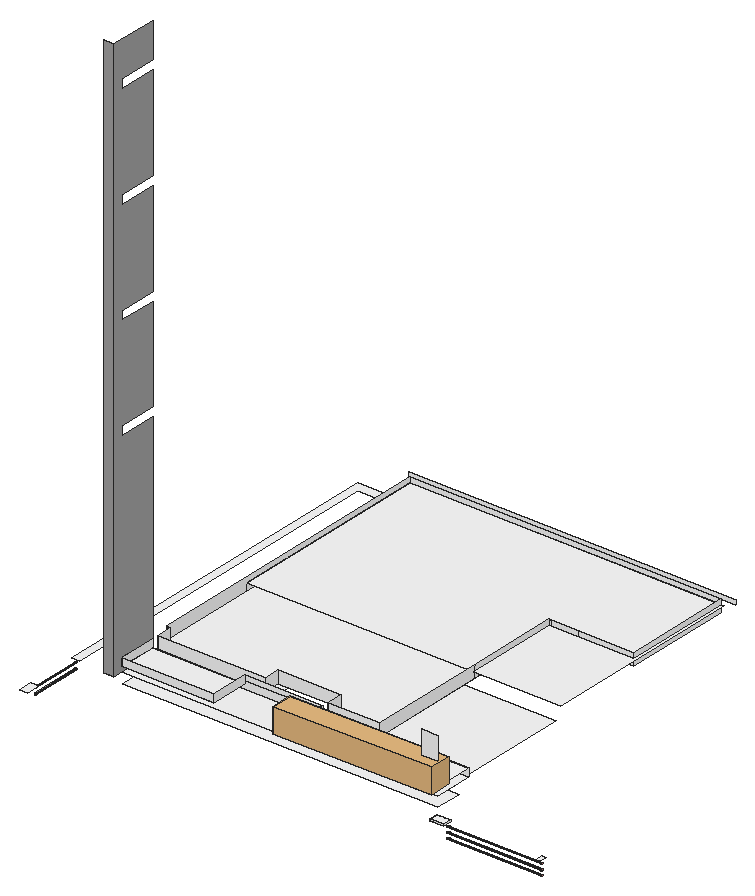
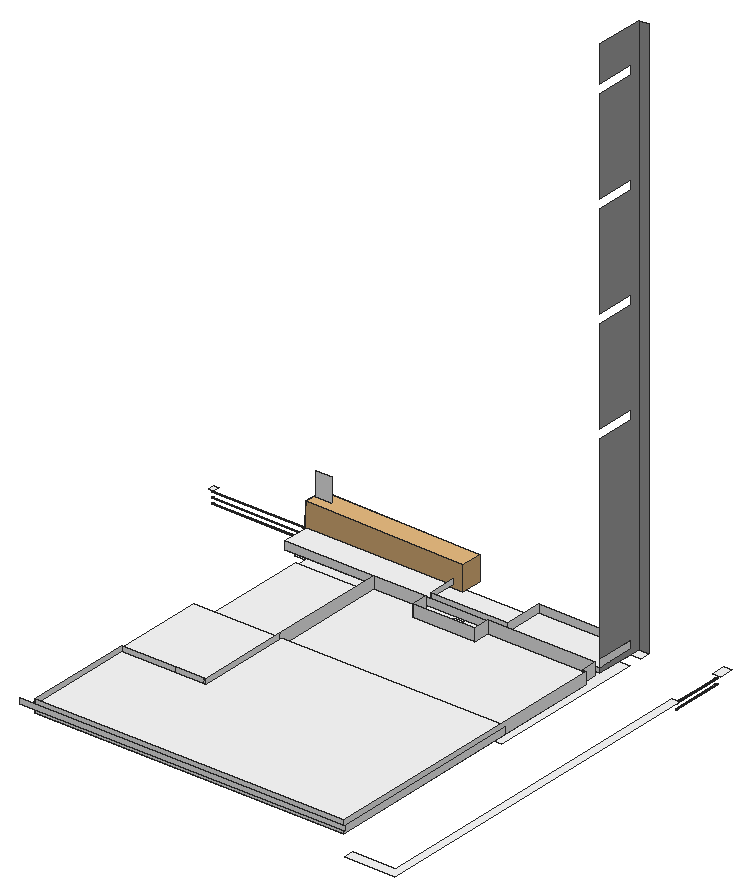
# SketchUp Ruby script. Lengths in inches.
U = 1.inch
M = Sketchup.active_model
def pt(a) = Geom::Point3d.new(a.map { |v| v * U })
def face(e, loops, mat)
  f = e.add_face(loops[0].map { |a| pt(a) })
  loops[1..].each { |l| e.add_face(l.map { |a| pt(a) }).erase! }
  f.material = f.back_material = mat if mat
  f
end
# faces: each face lists its corners as indices into pts; further lists are holes
def faces(e, pts, list, mat = nil) = list.each { |f| face(e, (f[0].is_a?(Array) ? f : [f]).map { |l| l.map { |i| pts[i] } }, mat) }
# xy, xz, yz: faces in a plane at the given z, y or x. An outline is a flat list of corners, or four numbers for a rectangle; further outlines are holes
def ring(l) = l.size == 4 ? [[l[0], l[1]], [l[2], l[1]], [l[2], l[3]], [l[0], l[3]]] : l.each_slice(2).to_a
def flat(e, list, mat, &to3) = list.each { |f| face(e, (f[0].is_a?(Array) ? f : [f]).map { |l| ring(l).map { |u, v| to3.(u, v) } }, mat) }
def xy(e, z, list, mat = nil) = flat(e, list, mat) { |x, y| [x, y, z] }
def xz(e, y, list, mat = nil) = flat(e, list, mat) { |x, z| [x, y, z] }
def yz(e, x, list, mat = nil) = flat(e, list, mat) { |y, z| [x, y, z] }
def lines(e, pts, list) = list.each { |a, b| e.add_line(pt(pts[a]), pt(pts[b])) }
# prism: a flat outline (further loops are holes) pulled along v
def prism(e, loops, v, mat = nil)
  f = face(e, loops, mat); d = Geom::Vector3d.new(v.map { |x| x * U })
  f.pushpull(f.normal.samedirection?(d) ? d.length : -d.length)
end
def box(e, o, s, mat = nil) = prism(e, [[o, [o[0] + s[0], o[1], o[2]], [o[0] + s[0], o[1] + s[1], o[2]], [o[0], o[1] + s[1], o[2]]]], [0, 0, s[2]], mat)
def at(x, y, z, deg = 0) = Geom::Transformation.translation(pt([x, y, z])) * Geom::Transformation.rotation(ORIGIN, Z_AXIS, deg.degrees)
def axes(o, x, y, z) = Geom::Transformation.new([*x, 0, *y, 0, *z, 0, *pt(o).to_a, 1])
def part(name) = M.definitions.add(name)
# library, detail: a bought-in or finely detailed component or shape, given as its bounding box
def library(name, o, s) = part(name).tap { |d| box(d.entities, o, s) }
def detail(e, o, s) = box(e.add_group.entities, o, s)
def put(e, d, t, mat = nil) = e.add_instance(d, t).tap { |i| i.material = mat if mat }
def group(e, t, mat = nil) = e.add_group.tap { |g| g.transformation = t; g.material = mat if mat }.entities
root = M.entities
M.materials.add("[Color M00]").color = [255, 255, 255]
M.materials.add("[Stone Vein Gray]").color = [166, 165, 165]
M.materials.add("[Tile Various Tan]").color = [221, 130, 130]
c1 = library("Living wall panel",[-0.54,-4.26,-5.13],[55.52,26.12,125.59])
xy(root,97.5625,[[0,21.25,9.51,37.7],[0,100.01,9.51,100.01,9.51,523,61.5,523,61.5,535.125,0,535.125]],"[Color M00]")
xy(root,103.5,[[468.6875,58.68,483.82,59.99],[483.82,58.68,485.57,59.99],[468.6875,59.99,469.1875,69.01],[469.1875,59.99,485.07,68.51],[485.07,59.99,485.57,69.01],
  [469.1875,68.51,483.82,69.01],[483.82,68.51,485.07,69.01],[74.88,83.25,74.88,279.08,203.28,279.08,203.28,105.8125,216.21,105.8125,216.21,125.75,251.02,125.75,251.02,115.3125,264.79,115.3125,264.79,129.875,445.32,129.875,445.32,115.3125,458.625,115.3125,458.625,83.25]],"[Color M00]")
xy(root,105.25,[[468.6875,58.68,485.57,69.01],[596.34,59.99,601.375,68.51]],"[Color M00]")
xy(root,106.9375,[[264.79,129.875,445.32,279.08]],"[Color M00]")
xy(root,116.25,[[61.5,71.125,73.74,83.25],[73.74,83.25,458.625,129.875]],"[Color M00]")
xy(root,116.6875,[[73.74,137.58,73.74,156.83,69.2,156.83,69.2,527.42,447.125,527.42,447.125,394.46,344.25,394.46,344.25,137.58,281.18,137.58,281.18,156.83,204.98,156.83,204.98,137.58]],"[Color M00]")
xy(root,121.875,[[73.74,83.25,186.35,129.875]],"[Color M00]")
xy(root,125.5625,[[281.18,83.25,458.625,129.875],[69.2,279.08,450.92,527.42]],"[Color M00]")
xz(root,58.68,[[468.6875,103.5,485.57,105.25]],"[Color M00]")
xz(root,69.01,[[468.6875,103.5,483.82,105.25],[483.82,103.5,485.57,105.25]],"[Color M00]")
xz(root,71.125,[[61.5,116.25,73.74,805.18]],"[Stone Vein Gray]")
xz(root,83.25,[[73.74,121.875,186.35,131.5625],[281.18,125.5625,458.625,125.5625,458.625,181.84,439.11,181.84,439.11,143.75,281.18,143.75]],"[Color M00]")
xz(root,129.875,[[264.79,103.5,445.32,106.9375],[73.74,116.25,458.625,116.25,458.625,125.5625,186.35,125.5625,186.35,121.875,73.74,121.875],[186.35,125.5625,281.18,131.5625]],"[Color M00]")
xz(root,137.58,[[73.74,116.6875,204.98,131.5625],[281.18,116.6875,344.25,131.5625]],"[Color M00]")
xz(root,156.83,[[69.2,116.6875,73.74,131.5625],[204.98,116.6875,281.18,131.5625]],"[Color M00]")
xz(root,394.46,[[344.25,116.6875,346.4375,131.5625],[346.4375,116.6875,381.25,131.5625],[381.25,116.6875,447.125,131.5625]],"[Color M00]")
xz(root,527.42,[[69.2,116.6875,447.125,125.5625],[69.2,125.5625,447.125,131.5625]],"[Color M00]")
xz(root,535.125,[[61.5,125.5625,458.625,131.5625]],"[Color M00]")
yz(root,4.15,[[37.7,87.41,100.01,87.6],[37.7,94.41,100.01,94.6]],"[Color M00]")
yz(root,69.2,[[156.83,116.6875,156.83,131.5625,527.42,131.5625,527.42,125.5625,279.08,125.5625,279.08,116.6875],[279.08,116.6875,527.42,125.5625]],"[Color M00]")
yz(root,73.74,[[137.58,116.6875,156.83,131.5625],[83.25,121.875,129.875,131.5625]],"[Color M00]")
yz(root,73.74,[[71.125,116.25,129.875,116.25,129.875,121.875,83.25,121.875,83.25,131.8125,129.875,131.8125,129.875,372.9375,83.25,372.9375,83.25,383.8125,129.875,383.8125,129.875,498.9375,83.25,498.9375,83.25,509.5625,129.875,509.5625,129.875,624.9375,83.25,624.9375,83.25,635.8125,129.875,635.8125,129.875,750.9375,83.25,750.9375,83.25,761.8125,129.875,761.8125,129.875,805.18,71.125,805.18]],"[Stone Vein Gray]")
yz(root,186.35,[[83.25,121.875,129.875,131.5625]],"[Color M00]")
yz(root,204.98,[[137.58,116.6875,156.83,131.5625]],"[Color M00]")
yz(root,281.18,[[137.58,116.6875,156.83,131.5625],[83.25,125.5625,83.25,143.75,91.3,143.75,91.3,131.5625,129.875,131.5625,129.875,125.5625]],"[Color M00]")
yz(root,344.25,[[137.58,116.6875,281.78,131.5625],[281.78,116.6875,394.46,131.5625]],"[Color M00]")
yz(root,447.125,[[394.46,116.6875,527.42,131.5625]],"[Color M00]")
yz(root,468.6875,[[58.68,103.5,69.01,105.25]],"[Color M00]")
yz(root,485.57,[[58.68,103.5,69.01,105.25]],"[Color M00]")
yz(root,601.375,[[63.79,86.97,63.95,87,64.1,87.06,64.23,87.16,64.33,87.29,64.39,87.4375,64.41,87.6,64.39,87.76,64.33,87.91,64.23,88.04,64.1,88.14,63.95,88.2,63.79,88.22,63.63,88.2,63.48,88.14,63.35,88.04,63.25,87.91,63.1875,87.76,63.16,87.6,63.1875,87.4375,63.25,87.29,63.35,87.16,63.48,87.06,63.63,87],[63.79,93.41,63.95,93.43,64.1,93.5,64.23,93.6,64.33,93.72,64.39,93.875,64.41,94.04,64.39,94.2,64.33,94.35,64.23,94.48,64.1,94.58,63.95,94.64,63.79,94.66,63.63,94.64,63.48,94.58,63.35,94.48,63.25,94.35,63.1875,94.2,63.16,94.04,63.1875,93.875,63.25,93.72,63.35,93.6,63.48,93.5,63.63,93.43],[63.79,100.29,63.95,100.31,64.1,100.37,64.23,100.47,64.33,100.6,64.39,100.75,64.41,100.91,64.39,101.07,64.33,101.22,64.23,101.35,64.1,101.45,63.95,101.52,63.79,101.54,63.63,101.52,63.48,101.45,63.35,101.35,63.25,101.22,63.1875,101.07,63.16,100.91,63.1875,100.75,63.25,100.6,63.35,100.47,63.48,100.37,63.63,100.31]],"[Tile Various Tan]")
p = [[4.46,100.01,86.92],[4.64,100.01,86.83],[4.64,37.7,86.83],[4.46,37.7,86.92],[4.83,100.01,86.79],[4.83,37.7,86.79],
  [5.02,100.01,86.8],[5.02,37.7,86.8],[5.21,100.01,86.86],[5.21,37.7,86.86],[4.32,100.01,87.05],[4.32,37.7,87.05],
  [5.375,100.01,86.96],[5.375,37.7,86.96],[5.51,100.01,87.11],[5.51,37.7,87.11],[485.07,63.48,87.06],[485.07,63.63,87],
  [601.375,63.63,87],[601.375,63.48,87.06],[485.07,63.79,86.97],[601.375,63.79,86.97],[485.07,63.95,87],[601.375,63.95,87],
  [485.07,64.1,87.06],[601.375,64.1,87.06],[4.21,100.01,87.22],[4.21,37.7,87.22],[5.6,100.01,87.28],[5.6,37.7,87.28],
  [485.07,63.35,87.16],[601.375,63.35,87.16],[485.07,64.23,87.16],[601.375,64.23,87.16],[4.15,100.01,87.41],[4.15,37.7,87.41],
  [485.07,63.25,87.29],[601.375,63.25,87.29],[485.07,64.33,87.29],[601.375,64.33,87.29],[5.64,100.01,87.47],[5.64,37.7,87.47],
  [485.07,63.1875,87.4375],[601.375,63.1875,87.4375],[485.07,64.39,87.4375],[601.375,64.39,87.4375],[485.07,63.16,87.6],[601.375,63.16,87.6],
  [485.07,64.41,87.6],[601.375,64.41,87.6],[5.63,100.01,87.67],[5.63,37.7,87.67],[4.1875,100.01,87.79],[4.15,100.01,87.6],
  [4.15,37.7,87.6],[4.1875,37.7,87.79],[485.07,63.1875,87.76],[601.375,63.1875,87.76],[485.07,64.39,87.76],[601.375,64.39,87.76],
  [5.57,100.01,87.85],[5.57,37.7,87.85],[4.28,100.01,87.97],[4.28,37.7,87.97],[485.07,63.25,87.91],[601.375,63.25,87.91],
  [485.07,64.33,87.91],[601.375,64.33,87.91],[5.47,100.01,88.02],[5.47,37.7,88.02],[485.07,63.35,88.04],[601.375,63.35,88.04],
  [485.07,64.23,88.04],[601.375,64.23,88.04],[4.41,100.01,88.11],[4.41,37.7,88.11],[5.32,100.01,88.15],[5.32,37.7,88.15],
  [485.07,63.48,88.14],[601.375,63.48,88.14],[485.07,64.1,88.14],[601.375,64.1,88.14],[4.58,100.01,88.22],[4.58,37.7,88.22],
  [485.07,63.63,88.2],[601.375,63.63,88.2],[485.07,63.95,88.2],[601.375,63.95,88.2],[4.76,100.01,88.27],[4.76,37.7,88.27],
  [5.15,100.01,88.24],[4.96,100.01,88.28],[4.96,37.7,88.28],[5.15,37.7,88.24],[485.07,63.79,88.22],[601.375,63.79,88.22],
  [485.07,63.48,93.5],[485.07,63.63,93.43],[601.375,63.63,93.43],[601.375,63.48,93.5],[485.07,63.79,93.41],[601.375,63.79,93.41],
  [485.07,63.95,93.43],[601.375,63.95,93.43],[485.07,64.1,93.5],[601.375,64.1,93.5],[485.07,63.35,93.6],[601.375,63.35,93.6],
  [485.07,64.23,93.6],[601.375,64.23,93.6],[485.07,63.25,93.72],[601.375,63.25,93.72],[485.07,64.33,93.72],[601.375,64.33,93.72],
  [485.07,63.1875,93.875],[601.375,63.1875,93.875],[485.07,64.39,93.875],[601.375,64.39,93.875],[4.46,100.01,93.92],[4.64,100.01,93.83],
  [4.64,37.7,93.83],[4.46,37.7,93.92],[4.83,100.01,93.79],[4.83,37.7,93.79],[5.02,100.01,93.8],[5.02,37.7,93.8],
  [5.21,100.01,93.86],[5.21,37.7,93.86],[4.32,100.01,94.05],[4.32,37.7,94.05],[5.375,100.01,93.96],[5.375,37.7,93.96],
  [485.07,63.16,94.04],[601.375,63.16,94.04],[485.07,64.41,94.04],[601.375,64.41,94.04],[5.51,100.01,94.11],[5.51,37.7,94.11],
  [485.07,63.1875,94.2],[601.375,63.1875,94.2],[485.07,64.39,94.2],[601.375,64.39,94.2],[4.21,100.01,94.22],[4.21,37.7,94.22],
  [5.6,100.01,94.28],[5.6,37.7,94.28],[4.15,100.01,94.41],[4.15,37.7,94.41],[485.07,63.25,94.35],[601.375,63.25,94.35],
  [485.07,64.33,94.35],[601.375,64.33,94.35],[5.64,100.01,94.47],[5.64,37.7,94.47],[485.07,63.35,94.48],[601.375,63.35,94.48],
  [485.07,64.23,94.48],[601.375,64.23,94.48],[5.63,100.01,94.67],[5.63,37.7,94.67],[485.07,63.48,94.58],[601.375,63.48,94.58],
  [485.07,64.1,94.58],[601.375,64.1,94.58],[4.1875,100.01,94.79],[4.15,100.01,94.6],[4.15,37.7,94.6],[4.1875,37.7,94.79],
  [485.07,63.63,94.64],[601.375,63.63,94.64],[485.07,63.79,94.66],[601.375,63.79,94.66],[485.07,63.95,94.64],[601.375,63.95,94.64],
  [5.57,100.01,94.85],[5.57,37.7,94.85],[4.28,100.01,94.97],[4.28,37.7,94.97],[5.47,100.01,95.02],[5.47,37.7,95.02],
  [4.41,100.01,95.11],[4.41,37.7,95.11],[5.32,100.01,95.15],[5.32,37.7,95.15],[4.58,100.01,95.22],[4.58,37.7,95.22],
  [4.76,100.01,95.27],[4.76,37.7,95.27],[5.15,100.01,95.24],[4.96,100.01,95.28],[4.96,37.7,95.28],[5.15,37.7,95.24],
  [485.07,63.48,100.37],[485.07,63.63,100.31],[601.375,63.63,100.31],[601.375,63.48,100.37],[485.07,63.79,100.29],[601.375,63.79,100.29],
  [485.07,63.95,100.31],[601.375,63.95,100.31],[485.07,64.1,100.37],[601.375,64.1,100.37],[485.07,63.35,100.47],[601.375,63.35,100.47],
  [485.07,64.23,100.47],[601.375,64.23,100.47],[485.07,63.25,100.6],[601.375,63.25,100.6],[485.07,64.33,100.6],[601.375,64.33,100.6],
  [485.07,63.1875,100.75],[601.375,63.1875,100.75],[485.07,64.39,100.75],[601.375,64.39,100.75],[485.07,63.16,100.91],[601.375,63.16,100.91],
  [485.07,64.41,100.91],[601.375,64.41,100.91],[485.07,63.1875,101.07],[601.375,63.1875,101.07],[485.07,64.39,101.07],[601.375,64.39,101.07],
  [485.07,63.25,101.22],[601.375,63.25,101.22],[485.07,64.33,101.22],[601.375,64.33,101.22],[485.07,63.35,101.35],[601.375,63.35,101.35],
  [485.07,64.23,101.35],[601.375,64.23,101.35],[485.07,63.48,101.45],[601.375,63.48,101.45],[485.07,64.1,101.45],[601.375,64.1,101.45],
  [485.07,63.63,101.52],[601.375,63.63,101.52],[485.07,63.79,101.54],[601.375,63.79,101.54],[485.07,63.95,101.52],[601.375,63.95,101.52],
  [73.74,129.875,116.25],[61.5,129.875,116.25]]
faces(root,p,[[0,1,2,3],[1,4,5,2],[4,6,7,5],[6,8,9,7],[10,0,3,11],[8,12,13,9],[12,14,15,13],[16,17,18,19],
  [17,20,21,18],[20,22,23,21],[22,24,25,23],[26,10,11,27],[14,28,29,15],[30,16,19,31],[24,32,33,25],[34,26,27,35],
  [36,30,31,37],[32,38,39,33],[28,40,41,29],[42,36,37,43],[38,44,45,39],[46,42,43,47],[44,48,49,45],[40,50,51,41],
  [52,53,54,55],[56,46,47,57],[48,58,59,49],[50,60,61,51],[62,52,55,63],[64,56,57,65],[58,66,67,59],[60,68,69,61],
  [70,64,65,71],[66,72,73,67],[74,62,63,75],[68,76,77,69],[78,70,71,79],[72,80,81,73],[82,74,75,83],[84,78,79,85],
  [80,86,87,81],[88,82,83,89],[90,91,92,93],[76,90,93,77],[94,84,85,95],[86,94,95,87],[91,88,89,92],[96,97,98,99],
  [97,100,101,98],[100,102,103,101],[102,104,105,103],[106,96,99,107],[104,108,109,105],[110,106,107,111],[108,112,113,109],[114,110,111,115],
  [112,116,117,113],[118,119,120,121],[119,122,123,120],[122,124,125,123],[124,126,127,125],[128,118,121,129],[126,130,131,127],[132,114,115,133],
  [116,134,135,117],[130,136,137,131],[138,132,133,139],[134,140,141,135],[142,128,129,143],[136,144,145,137],[146,142,143,147],[148,138,139,149],
  [140,150,151,141],[144,152,153,145],[154,148,149,155],[150,156,157,151],[152,158,159,153],[160,154,155,161],[156,162,163,157],[164,165,166,167],
  [168,160,161,169],[170,168,169,171],[172,170,171,173],[162,172,173,163],[158,174,175,159],[176,164,167,177],[174,178,179,175],[180,176,177,181],
  [178,182,183,179],[184,180,181,185],[186,184,185,187],[188,189,190,191],[182,188,191,183],[189,186,187,190],[192,193,194,195],[193,196,197,194],
  [196,198,199,197],[198,200,201,199],[202,192,195,203],[200,204,205,201],[206,202,203,207],[204,208,209,205],[210,206,207,211],[208,212,213,209],
  [214,210,211,215],[212,216,217,213],[218,214,215,219],[216,220,221,217],[222,218,219,223],[220,224,225,221],[226,222,223,227],[224,228,229,225],
  [230,226,227,231],[228,232,233,229],[234,230,231,235],[236,234,235,237],[238,236,237,239],[232,238,239,233]],"[Color M00]")
lines(root,p,[[240,241]])
put(root,c1,axes([275.83,74.53,151.66],[0.0058,0,-0.53997],[0,1,0],[1.53606,0,0.0165]),"[Color M00]")
